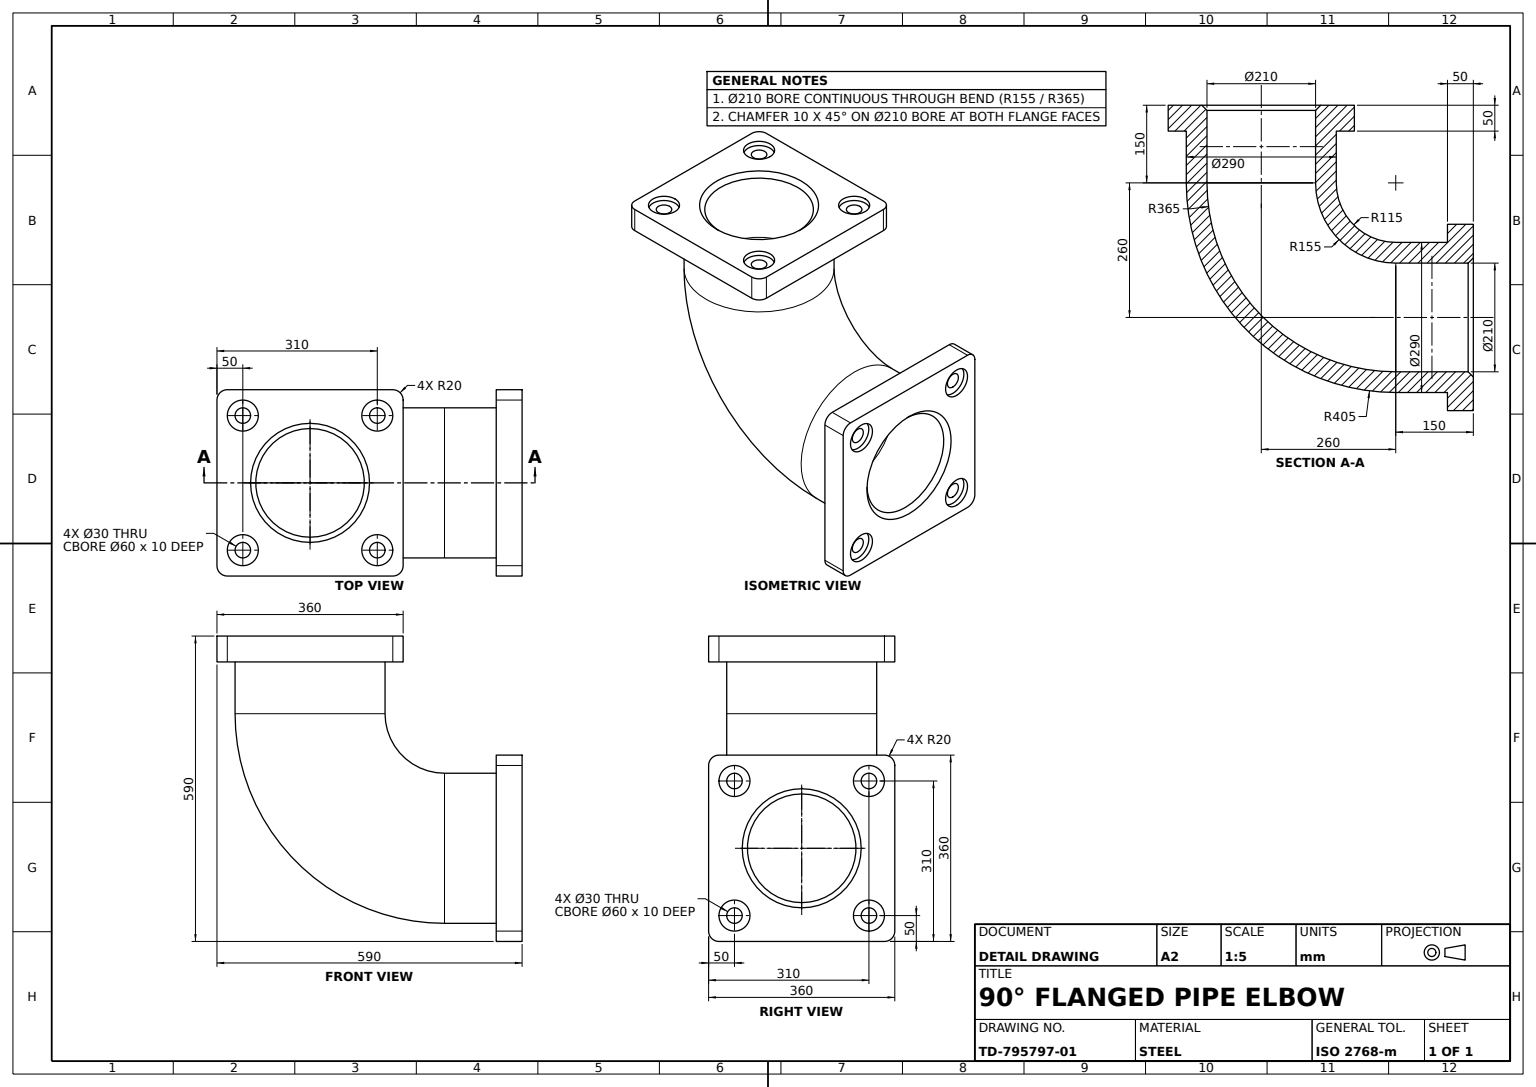
solid
v1 (-310,400,130)
v2 (-250,400,130)
e1 v1 v2 CIRCLE(AX(P(-280,400,130),D(0,1,0),D(1,0,0)),30)
e2 v2 v1 CIRCLE(AX(P(-280,400,130),D(0,1,0),D(1,0,0)),30)
v3 (-265,400,130)
v4 (-295,400,130)
e3 v3 v4 CIRCLE(AX(P(-280,400,130),D(0,1,0),D(1,0,0)),15)
e4 v4 v3 CIRCLE(AX(P(-280,400,130),D(0,1,0),D(1,0,0)),15)
face PLANE(AX(P(-280,400,130),D(0,1,0),D(1,0,0))) [e1 e2] [-e3 -e4]
v5 (-50,-145,-130)
v6 (-50,-115,-130)
e5 v5 v6 CIRCLE(AX(P(-50,-130,-130),D(-1,0,0),D(0,0,-1)),15)
v7 (-10,-115,-130)
e6 v6 v7 LINE
v8 (-10,-145,-130)
e7 v7 v8 CIRCLE(AX(P(-10,-130,-130),D(1,0,0),D(0,0,1)),15)
e8 v5 v8 LINE
face CYL(AX(P(-590.001,-130,-130),D(1,0,0),D(0,1,0)),15) rev [e5 e6 e7 -e8]
v9 (-590,410,-160)
v10 (-590,360,-160)
e9 v9 v10 LINE
v11 (-590,360,160)
e10 v10 v11 LINE
v12 (-590,410,160)
e11 v11 v12 LINE
e12 v9 v12 LINE
face PLANE(AX(P(-590,360,0),D(-1,0,0),D(0,-1,0))) [e9 e10 e11 -e12]
v13 (-510,400,-130)
v14 (-570,400,-130)
e13 v13 v14 CIRCLE(AX(P(-540,400,-130),D(0,1,0),D(-1,0,0)),30)
v15 (-510,410,-130)
e14 v13 v15 LINE
v16 (-570,410,-130)
e15 v15 v16 CIRCLE(AX(P(-540,410,-130),D(0,1,0),D(-1,0,0)),30)
e16 v14 v16 LINE
face CYL(AX(P(-540,400,-130),D(0,1,0),D(-1,0,0)),30) rev [-e13 e14 e15 -e16]
v17 (-555,360,-130)
v18 (-555,400,-130)
e17 v17 v18 LINE
v19 (-525,360,-130)
e18 v17 v19 CIRCLE(AX(P(-540,360,-130),D(0,-1,0),D(-1,0,0)),15)
v20 (-525,400,-130)
e19 v19 v20 LINE
e20 v20 v18 CIRCLE(AX(P(-540,400,-130),D(0,1,0),D(-1,0,0)),15)
face CYL(AX(P(-540,-180.001,-130),D(0,1,0),D(-1,0,0)),15) rev [-e17 e18 e19 e20]
e21 v16 v15 CIRCLE(AX(P(-540,410,-130),D(0,1,0),D(-1,0,0)),30)
e22 v14 v13 CIRCLE(AX(P(-540,400,-130),D(0,1,0),D(-1,0,0)),30)
face CYL(AX(P(-540,400,-130),D(0,1,0),D(-1,0,0)),30) rev [e16 e21 -e14 -e22]
v21 (-50,145,0)
v22 (-150,145,0)
e23 v21 v22 LINE
v23 (-50,-145,0)
e24 v23 v21 CIRCLE(AX(P(-50,0,0),D(1,0,0),D(0,0,-1)),145)
v24 (-150,-145,0)
e25 v23 v24 LINE
e26 v24 v22 CIRCLE(AX(P(-150,0,0),D(1,0,0),D(0,0,-1)),145)
face CYL(AX(P(0,0,0),D(-1,0,0),D(0,-1,0)),145) [-e23 -e24 e25 e26]
v25 (-280,400,-100)
v26 (-280,410,-100)
e27 v25 v26 LINE
v27 (-280,410,-160)
e28 v26 v27 CIRCLE(AX(P(-280,410,-130),D(0,1,0),D(0,0,-1)),30)
v28 (-280,400,-160)
e29 v28 v27 LINE
e30 v25 v28 CIRCLE(AX(P(-280,400,-130),D(0,1,0),D(0,0,-1)),30)
face CYL(AX(P(-280,400,-130),D(0,1,0),D(0,0,1)),30) rev [e27 e28 -e29 -e30]
v29 (-150,-105,0)
v30 (-150,105,0)
e31 v29 v30 CIRCLE(AX(P(-150,0,0),D(1,0,0),D(0,-1,0)),105)
v31 (-305,260,0)
e32 v30 v31 CIRCLE(AX(P(-150,260,0),D(0,0,-1),D(-1,0,0)),155)
v32 (-410,260,-105)
e33 v32 v31 CIRCLE(AX(P(-410,260,0),D(0,-1,0),D(0,0,-1)),105)
v33 (-515,260,0)
e34 v33 v32 CIRCLE(AX(P(-410,260,0),D(0,-1,0),D(0,0,-1)),105)
e35 v29 v33 CIRCLE(AX(P(-150,260,0),D(0,0,-1),D(-1,0,0)),365)
face TORUS(AX(P(-150,260,0),D(0,0,-1),D(-1,0,0)),260,105) rev [e31 e32 -e33 -e34 -e35]
v34 (-250,360,180)
v35 (-250,410,180)
e36 v34 v35 LINE
v36 (-230,360,160)
e37 v36 v34 CIRCLE(AX(P(-250,360,160),D(0,-1,0),D(-1,0,0)),20)
v37 (-230,410,160)
e38 v37 v36 LINE
e39 v35 v37 CIRCLE(AX(P(-250,410,160),D(0,1,0),D(1,0,0)),20)
face CYL(AX(P(-250,360,160),D(0,-1,0),D(1,0,0)),20) [-e36 -e37 -e38 -e39]
v38 (-10,-105,0)
e40 v38 v29 LINE
v39 (-10,105,0)
e41 v38 v39 CIRCLE(AX(P(-10,0,0),D(1,0,0),D(0,1,0)),105)
e42 v39 v30 LINE
face CYL(AX(P(0,0,0),D(-1,0,0),D(0,-1,0)),105) rev [-e31 -e40 e41 e42]
v40 (-540,360,115)
v41 (-540,360,145)
e43 v40 v41 CIRCLE(AX(P(-540,360,130),D(0,-1,0),D(-1,0,0)),15)
v42 (-540,400,145)
e44 v41 v42 LINE
v43 (-540,400,115)
e45 v42 v43 CIRCLE(AX(P(-540,400,130),D(0,1,0),D(0,0,1)),15)
e46 v40 v43 LINE
face CYL(AX(P(-540,-180.001,130),D(0,1,0),D(0,0,1)),15) rev [e43 e44 e45 -e46]
v44 (-280,360,-115)
v45 (-280,400,-115)
e47 v44 v45 LINE
v46 (-280,400,-145)
e48 v45 v46 CIRCLE(AX(P(-280,400,-130),D(0,1,0),D(0,0,-1)),15)
v47 (-280,360,-145)
e49 v47 v46 LINE
e50 v47 v44 CIRCLE(AX(P(-280,360,-130),D(0,-1,0),D(-1,0,0)),15)
face CYL(AX(P(-280,-180.001,-130),D(0,1,0),D(0,0,1)),15) rev [e47 e48 -e49 e50]
v48 (0,-160,180)
v49 (0,-180,160)
e51 v48 v49 CIRCLE(AX(P(0,-160,160),D(1,0,0),D(0,0,-1)),20)
v50 (-50,-160,180)
e52 v50 v48 LINE
v51 (-50,-180,160)
e53 v51 v50 CIRCLE(AX(P(-50,-160,160),D(-1,0,0),D(0,0,-1)),20)
e54 v49 v51 LINE
face CYL(AX(P(-50,-160,160),D(1,0,0),D(0,0,-1)),20) [-e51 -e52 -e53 -e54]
e55 v30 v29 CIRCLE(AX(P(-150,0,0),D(1,0,0),D(0,-1,0)),105)
v52 (-410,260,105)
e56 v52 v33 CIRCLE(AX(P(-410,260,0),D(0,-1,0),D(0,0,-1)),105)
e57 v31 v52 CIRCLE(AX(P(-410,260,0),D(0,-1,0),D(0,0,-1)),105)
face TORUS(AX(P(-150,260,0),D(0,0,-1),D(-1,0,0)),260,105) rev [e55 e35 -e56 -e57 -e32]
v53 (-295,360,130)
v54 (-265,360,130)
e58 v53 v54 CIRCLE(AX(P(-280,360,130),D(0,-1,0),D(-1,0,0)),15)
e59 v54 v3 LINE
e60 v53 v4 LINE
face CYL(AX(P(-280,-180.001,130),D(0,1,0),D(-1,0,0)),15) rev [e58 e59 e3 -e60]
v55 (0,100,-130)
v56 (0,160,-130)
e61 v55 v56 CIRCLE(AX(P(0,130,-130),D(1,0,0),D(0,-1,0)),30)
v57 (-10,160,-130)
e62 v57 v56 LINE
v58 (-10,100,-130)
e63 v58 v57 CIRCLE(AX(P(-10,130,-130),D(1,0,0),D(0,-1,0)),30)
e64 v58 v55 LINE
face CYL(AX(P(-10,130,-130),D(1,0,0),D(0,1,0)),30) rev [e61 -e62 -e63 e64]
v59 (-570,410,180)
e65 v59 v35 LINE
v60 (-570,360,180)
e66 v59 v60 LINE
e67 v60 v34 LINE
face PLANE(AX(P(0,360,180),D(0,0,1),D(1,0,0))) [e36 -e65 e66 e67]
v61 (-50,115,-130)
v62 (-50,145,-130)
e68 v61 v62 CIRCLE(AX(P(-50,130,-130),D(-1,0,0),D(0,0,-1)),15)
e69 v62 v61 CIRCLE(AX(P(-50,130,-130),D(-1,0,0),D(0,0,-1)),15)
e70 v21 v23 CIRCLE(AX(P(-50,0,0),D(1,0,0),D(0,0,-1)),145)
e71 v6 v5 CIRCLE(AX(P(-50,-130,-130),D(-1,0,0),D(0,0,-1)),15)
v63 (-50,-160,-180)
v64 (-50,-180,-160)
e72 v63 v64 CIRCLE(AX(P(-50,-160,-160),D(-1,0,0),D(0,0,-1)),20)
e73 v51 v64 LINE
v65 (-50,160,180)
e74 v65 v50 LINE
v66 (-50,180,160)
e75 v65 v66 CIRCLE(AX(P(-50,160,160),D(-1,0,0),D(0,0,-1)),20)
v67 (-50,180,-160)
e76 v66 v67 LINE
v68 (-50,160,-180)
e77 v67 v68 CIRCLE(AX(P(-50,160,-160),D(-1,0,0),D(0,0,-1)),20)
e78 v68 v63 LINE
v69 (-50,130,115)
v70 (-50,130,145)
e79 v69 v70 CIRCLE(AX(P(-50,130,130),D(-1,0,0),D(0,0,-1)),15)
e80 v70 v69 CIRCLE(AX(P(-50,130,130),D(-1,0,0),D(0,0,-1)),15)
v71 (-50,-130,145)
v72 (-50,-130,115)
e81 v71 v72 CIRCLE(AX(P(-50,-130,130),D(-1,0,0),D(0,0,-1)),15)
e82 v72 v71 CIRCLE(AX(P(-50,-130,130),D(-1,0,0),D(0,0,-1)),15)
face PLANE(AX(P(-50,0,0),D(1,0,0),D(0,0,-1))) rev [-e68 -e69] [e24 e70] [-e5 -e71] [e72 -e73 e53 -e74 e75 e76 e77 e78] [-e79 -e80] [-e81 -e82]
e83 v60 v11 CIRCLE(AX(P(-570,360,160),D(0,-1,0),D(-1,0,0)),20)
e84 v12 v59 CIRCLE(AX(P(-570,410,160),D(0,1,0),D(1,0,0)),20)
face CYL(AX(P(-570,360,160),D(0,1,0),D(-1,0,0)),20) [-e11 -e83 -e66 -e84]
v73 (-570,360,-180)
e85 v10 v73 CIRCLE(AX(P(-570,360,-160),D(0,-1,0),D(-1,0,0)),20)
v74 (-570,410,-180)
e86 v74 v9 CIRCLE(AX(P(-570,410,-160),D(0,1,0),D(1,0,0)),20)
e87 v73 v74 LINE
face CYL(AX(P(-570,360,-160),D(0,-1,0),D(1,0,0)),20) [-e85 -e9 -e86 -e87]
v75 (-10,130,100)
v76 (-10,130,160)
e88 v75 v76 CIRCLE(AX(P(-10,130,130),D(1,0,0),D(0,0,-1)),30)
v77 (0,130,100)
e89 v75 v77 LINE
v78 (0,130,160)
e90 v77 v78 CIRCLE(AX(P(0,130,130),D(1,0,0),D(0,0,-1)),30)
e91 v76 v78 LINE
face CYL(AX(P(-10,130,130),D(1,0,0),D(0,0,-1)),30) rev [-e88 e89 e90 -e91]
v79 (-10,145,-130)
e92 v62 v79 LINE
v80 (-10,115,-130)
e93 v61 v80 LINE
e94 v80 v79 CIRCLE(AX(P(-10,130,-130),D(1,0,0),D(0,-1,0)),15)
face CYL(AX(P(-590.001,130,-130),D(1,0,0),D(0,1,0)),15) rev [-e92 e69 e93 e94]
e95 v44 v47 CIRCLE(AX(P(-280,360,-130),D(0,-1,0),D(-1,0,0)),15)
e96 v46 v45 CIRCLE(AX(P(-280,400,-130),D(0,1,0),D(0,0,-1)),15)
face CYL(AX(P(-280,-180.001,-130),D(0,1,0),D(0,0,1)),15) rev [-e47 e95 e49 e96]
v81 (0,-130,100)
v82 (0,-130,160)
e97 v81 v82 CIRCLE(AX(P(0,-130,130),D(1,0,0),D(0,1,0)),30)
v83 (-10,-130,160)
e98 v83 v82 LINE
v84 (-10,-130,100)
e99 v84 v83 CIRCLE(AX(P(-10,-130,130),D(1,0,0),D(0,1,0)),30)
e100 v84 v81 LINE
face CYL(AX(P(-10,-130,130),D(1,0,0),D(0,0,-1)),30) rev [e97 -e98 -e99 e100]
v85 (0,160,-180)
v86 (0,-160,-180)
e101 v85 v86 LINE
e102 v86 v63 LINE
e103 v68 v85 LINE
face PLANE(AX(P(-50,0,-180),D(0,0,1),D(0,-1,0))) rev [e101 e102 -e78 e103]
v87 (0,-115,0)
e104 v38 v87 LINE
e105 v39 v38 CIRCLE(AX(P(-10,0,0),D(1,0,0),D(0,1,0)),105)
v88 (0,115,0)
e106 v39 v88 LINE
e107 v87 v88 CIRCLE(AX(P(0,0,0),D(-1,0,0),D(0,0,-1)),115)
face CONE(AX(P(-10,0,0),D(1,0,0),D(0,1,0)),105,0.785398163) rev [-e104 -e105 e106 -e107]
e108 v19 v17 CIRCLE(AX(P(-540,360,-130),D(0,-1,0),D(-1,0,0)),15)
e109 v18 v20 CIRCLE(AX(P(-540,400,-130),D(0,1,0),D(-1,0,0)),15)
face CYL(AX(P(-540,-180.001,-130),D(0,1,0),D(-1,0,0)),15) rev [e108 e17 e109 -e19]
v89 (0,-160,-130)
v90 (0,-100,-130)
e110 v89 v90 CIRCLE(AX(P(0,-130,-130),D(1,0,0),D(0,0,1)),30)
v91 (-10,-100,-130)
e111 v91 v90 LINE
v92 (-10,-160,-130)
e112 v92 v91 CIRCLE(AX(P(-10,-130,-130),D(1,0,0),D(0,0,1)),30)
e113 v92 v89 LINE
face CYL(AX(P(-10,-130,-130),D(1,0,0),D(0,1,0)),30) rev [e110 -e111 -e112 e113]
e114 v8 v7 CIRCLE(AX(P(-10,-130,-130),D(1,0,0),D(0,0,1)),15)
face CYL(AX(P(-590.001,-130,-130),D(1,0,0),D(0,1,0)),15) rev [-e6 e71 e8 e114]
v93 (-410,260,-145)
v94 (-410,360,-145)
e115 v93 v94 LINE
v95 (-410,360,145)
e116 v95 v94 CIRCLE(AX(P(-410,360,0),D(0,1,0),D(-1,0,0)),145)
v96 (-410,260,145)
e117 v96 v95 LINE
v97 (-265,260,0)
e118 v97 v96 CIRCLE(AX(P(-410,260,0),D(0,-1,0),D(0,0,-1)),145)
e119 v93 v97 CIRCLE(AX(P(-410,260,0),D(0,-1,0),D(0,0,-1)),145)
face CYL(AX(P(-410,260,0),D(0,1,0),D(0,0,1)),145) [e115 -e116 -e117 -e118 -e119]
e120 v54 v53 CIRCLE(AX(P(-280,360,130),D(0,-1,0),D(-1,0,0)),15)
face CYL(AX(P(-280,-180.001,130),D(0,1,0),D(-1,0,0)),15) rev [-e59 e120 e60 e4]
v98 (-230,360,-160)
e121 v98 v36 LINE
v99 (-230,410,-160)
e122 v98 v99 LINE
e123 v99 v37 LINE
face PLANE(AX(P(-230,360,0),D(-1,0,0),D(0,0,1))) rev [e38 -e121 e122 e123]
e124 v91 v92 CIRCLE(AX(P(-10,-130,-130),D(1,0,0),D(0,0,1)),30)
e125 v90 v89 CIRCLE(AX(P(0,-130,-130),D(1,0,0),D(0,0,1)),30)
face CYL(AX(P(-10,-130,-130),D(1,0,0),D(0,1,0)),30) rev [-e124 e111 e125 -e113]
v100 (-555,260,0)
e126 v100 v93 CIRCLE(AX(P(-410,260,0),D(0,-1,0),D(0,0,-1)),145)
e127 v22 v97 CIRCLE(AX(P(-150,260,0),D(0,0,-1),D(-1,0,0)),115)
e128 v24 v100 CIRCLE(AX(P(-150,260,0),D(0,0,-1),D(-1,0,0)),405)
face TORUS(AX(P(-150,260,0),D(0,0,-1),D(-1,0,0)),260,145) [e126 e119 -e127 -e26 e128]
v101 (-250,410,130)
v102 (-310,410,130)
e129 v101 v102 CIRCLE(AX(P(-280,410,130),D(0,1,0),D(1,0,0)),30)
e130 v1 v102 LINE
e131 v2 v101 LINE
face CYL(AX(P(-280,400,130),D(0,1,0),D(-1,0,0)),30) rev [e129 -e130 -e2 e131]
e132 v22 v24 CIRCLE(AX(P(-150,0,0),D(1,0,0),D(0,0,-1)),145)
face CYL(AX(P(0,0,0),D(-1,0,0),D(0,-1,0)),145) [e23 e132 -e25 -e70]
e133 v41 v40 CIRCLE(AX(P(-540,360,130),D(0,-1,0),D(-1,0,0)),15)
e134 v43 v42 CIRCLE(AX(P(-540,400,130),D(0,1,0),D(0,0,1)),15)
face CYL(AX(P(-540,-180.001,130),D(0,1,0),D(0,0,1)),15) rev [e133 e46 e134 -e44]
face CYL(AX(P(0,0,0),D(-1,0,0),D(0,-1,0)),105) rev [-e42 e105 e40 -e55]
face PLANE(AX(P(-540,400,-130),D(0,1,0),D(-1,0,0))) [e22 e13] [-e20 -e109]
v103 (0,160,180)
e135 v103 v65 LINE
v104 (0,180,160)
e136 v104 v103 CIRCLE(AX(P(0,160,160),D(1,0,0),D(0,0,-1)),20)
e137 v66 v104 LINE
face CYL(AX(P(-50,160,160),D(-1,0,0),D(0,0,1)),20) [-e135 -e136 -e137 -e75]
v105 (0,180,-160)
e138 v105 v67 LINE
e139 v104 v105 LINE
face PLANE(AX(P(-50,180,0),D(0,-1,0),D(0,0,-1))) rev [e138 -e76 e137 e139]
e140 v76 v75 CIRCLE(AX(P(-10,130,130),D(1,0,0),D(0,0,-1)),30)
v106 (-10,130,145)
v107 (-10,130,115)
e141 v106 v107 CIRCLE(AX(P(-10,130,130),D(1,0,0),D(0,0,-1)),15)
e142 v107 v106 CIRCLE(AX(P(-10,130,130),D(1,0,0),D(0,0,-1)),15)
face PLANE(AX(P(-10,130,130),D(1,0,0),D(0,0,-1))) [e88 e140] [-e141 -e142]
v108 (-410,400,-105)
v109 (-410,400,105)
e143 v108 v109 CIRCLE(AX(P(-410,400,0),D(0,1,0),D(0,0,-1)),105)
v110 (-410,410,-115)
e144 v108 v110 LINE
v111 (-410,410,115)
e145 v111 v110 CIRCLE(AX(P(-410,410,0),D(0,-1,0),D(1,0,0)),115)
e146 v109 v111 LINE
face CONE(AX(P(-410,410,0),D(0,1,0),D(0,0,1)),115,0.785398163) rev [-e143 e144 -e145 -e146]
e147 v83 v84 CIRCLE(AX(P(-10,-130,130),D(1,0,0),D(0,1,0)),30)
e148 v82 v81 CIRCLE(AX(P(0,-130,130),D(1,0,0),D(0,1,0)),30)
face CYL(AX(P(-10,-130,130),D(1,0,0),D(0,0,-1)),30) rev [-e100 -e147 e98 e148]
e149 v96 v100 CIRCLE(AX(P(-410,260,0),D(0,-1,0),D(0,0,-1)),145)
face TORUS(AX(P(-150,260,0),D(0,0,-1),D(-1,0,0)),260,145) [e118 e149 -e128 -e132 e127]
v112 (0,-180,-160)
e150 v49 v112 LINE
e151 v64 v112 LINE
face PLANE(AX(P(-50,-180,0),D(0,-1,0),D(0,0,-1))) [-e150 e54 e73 e151]
v113 (-10,-130,145)
v114 (-10,-130,115)
e152 v113 v114 CIRCLE(AX(P(-10,-130,130),D(1,0,0),D(0,1,0)),15)
e153 v72 v114 LINE
e154 v71 v113 LINE
face CYL(AX(P(-590.001,-130,130),D(1,0,0),D(0,0,-1)),15) rev [e152 -e153 e82 e154]
e155 v79 v80 CIRCLE(AX(P(-10,130,-130),D(1,0,0),D(0,-1,0)),15)
e156 v57 v58 CIRCLE(AX(P(-10,130,-130),D(1,0,0),D(0,-1,0)),30)
face PLANE(AX(P(-10,130,-130),D(1,0,0),D(0,-1,0))) [-e155 -e94] [e156 e63]
e157 v52 v109 LINE
e158 v32 v108 LINE
face CYL(AX(P(-410,260,0),D(0,1,0),D(0,0,1)),105) rev [e143 -e157 e56 e34 e158]
e159 v88 v87 CIRCLE(AX(P(0,0,0),D(-1,0,0),D(0,0,-1)),115)
face CONE(AX(P(-10,0,0),D(1,0,0),D(0,1,0)),105,0.785398163) rev [-e106 -e41 e104 -e159]
e160 v109 v108 CIRCLE(AX(P(-410,400,0),D(0,1,0),D(0,0,-1)),105)
e161 v110 v111 CIRCLE(AX(P(-410,410,0),D(0,-1,0),D(1,0,0)),115)
face CONE(AX(P(-410,410,0),D(0,1,0),D(0,0,1)),115,0.785398163) rev [-e160 e146 -e161 -e144]
e162 v78 v77 CIRCLE(AX(P(0,130,130),D(1,0,0),D(0,0,-1)),30)
face CYL(AX(P(-10,130,130),D(1,0,0),D(0,0,-1)),30) rev [e91 e162 -e89 -e140]
e163 v94 v95 CIRCLE(AX(P(-410,360,0),D(0,1,0),D(-1,0,0)),145)
face CYL(AX(P(-410,260,0),D(0,1,0),D(0,0,1)),145) [-e126 -e149 e117 -e163 -e115]
e164 v28 v25 CIRCLE(AX(P(-280,400,-130),D(0,1,0),D(0,0,-1)),30)
face PLANE(AX(P(-280,400,-130),D(0,1,0),D(0,0,-1))) [e30 e164] [-e96 -e48]
v115 (-540,400,160)
v116 (-540,410,160)
e165 v115 v116 LINE
v117 (-540,400,100)
e166 v117 v115 CIRCLE(AX(P(-540,400,130),D(0,1,0),D(0,0,1)),30)
v118 (-540,410,100)
e167 v117 v118 LINE
e168 v118 v116 CIRCLE(AX(P(-540,410,130),D(0,1,0),D(0,0,1)),30)
face CYL(AX(P(-540,400,130),D(0,1,0),D(0,0,1)),30) rev [-e165 -e166 e167 e168]
e169 v56 v55 CIRCLE(AX(P(0,130,-130),D(1,0,0),D(0,-1,0)),30)
face CYL(AX(P(-10,130,-130),D(1,0,0),D(0,1,0)),30) rev [e62 e169 -e64 -e156]
e170 v27 v26 CIRCLE(AX(P(-280,410,-130),D(0,1,0),D(0,0,-1)),30)
e171 v116 v118 CIRCLE(AX(P(-540,410,130),D(0,1,0),D(0,0,1)),30)
e172 v102 v101 CIRCLE(AX(P(-280,410,130),D(0,1,0),D(1,0,0)),30)
v119 (-250,410,-180)
e173 v99 v119 CIRCLE(AX(P(-250,410,-160),D(0,1,0),D(1,0,0)),20)
e174 v74 v119 LINE
face PLANE(AX(P(-410,410,0),D(0,-1,0),D(0,0,-1))) rev [-e170 -e28] [-e171 -e168] [-e21 -e15] [-e172 -e129] [e161 e145] [e173 -e174 e86 e12 e84 e65 e39 -e123]
e175 v114 v113 CIRCLE(AX(P(-10,-130,130),D(1,0,0),D(0,1,0)),15)
face CYL(AX(P(-590.001,-130,130),D(1,0,0),D(0,0,-1)),15) rev [e175 -e154 e81 e153]
e176 v112 v86 CIRCLE(AX(P(0,-160,-160),D(1,0,0),D(0,0,-1)),20)
face CYL(AX(P(-50,-160,-160),D(-1,0,0),D(0,0,1)),20) [-e151 -e72 -e102 -e176]
e177 v115 v117 CIRCLE(AX(P(-540,400,130),D(0,1,0),D(0,0,1)),30)
face PLANE(AX(P(-540,400,130),D(0,1,0),D(0,0,1))) [-e134 -e45] [e166 e177]
v120 (-250,360,-180)
e178 v119 v120 LINE
e179 v73 v120 LINE
face PLANE(AX(P(0,360,-180),D(0,0,1),D(1,0,0))) rev [e178 -e179 e87 e174]
e180 v70 v106 LINE
e181 v69 v107 LINE
face CYL(AX(P(-590.001,130,130),D(1,0,0),D(0,0,-1)),15) rev [e180 e141 -e181 e79]
e182 v120 v98 CIRCLE(AX(P(-250,360,-160),D(0,-1,0),D(-1,0,0)),20)
face CYL(AX(P(-250,360,-160),D(0,1,0),D(-1,0,0)),20) [-e178 -e173 -e122 -e182]
face CYL(AX(P(-280,400,130),D(0,1,0),D(-1,0,0)),30) rev [e130 e172 -e131 -e1]
e183 v103 v48 LINE
e184 v85 v105 CIRCLE(AX(P(0,160,-160),D(1,0,0),D(0,0,-1)),20)
face PLANE(AX(P(0,0,0),D(1,0,0),D(0,0,-1))) [e159 e107] [e183 e51 e150 e176 -e101 e184 -e139 e136] [-e90 -e162] [-e125 -e110] [-e148 -e97] [-e61 -e169]
face PLANE(AX(P(-50,0,180),D(0,0,1),D(0,-1,0))) [e135 e74 e52 -e183]
face PLANE(AX(P(0,360,0),D(0,1,0),D(-1,0,0))) rev [-e50 -e95] [e163 e116] [-e18 -e108] [-e133 -e43] [-e67 e83 -e10 e85 e179 e182 e121 e37] [-e58 -e120]
face CYL(AX(P(-50,160,-160),D(1,0,0),D(0,0,-1)),20) [-e184 -e103 -e77 -e138]
face PLANE(AX(P(-10,-130,-130),D(1,0,0),D(0,0,1))) [e124 e112] [-e7 -e114]
face CYL(AX(P(-410,260,0),D(0,1,0),D(0,0,1)),105) rev [e160 -e158 e33 e57 e157]
face CYL(AX(P(-280,400,-130),D(0,1,0),D(0,0,1)),30) rev [e29 e170 -e27 -e164]
face CYL(AX(P(-590.001,130,130),D(1,0,0),D(0,0,-1)),15) rev [e80 e181 e142 -e180]
face CYL(AX(P(-540,400,130),D(0,1,0),D(0,0,1)),30) rev [e171 -e167 -e177 e165]
face CYL(AX(P(-590.001,130,-130),D(1,0,0),D(0,1,0)),15) rev [e155 -e93 e68 e92]
face PLANE(AX(P(-10,-130,130),D(1,0,0),D(0,1,0))) [e147 e99] [-e152 -e175]
